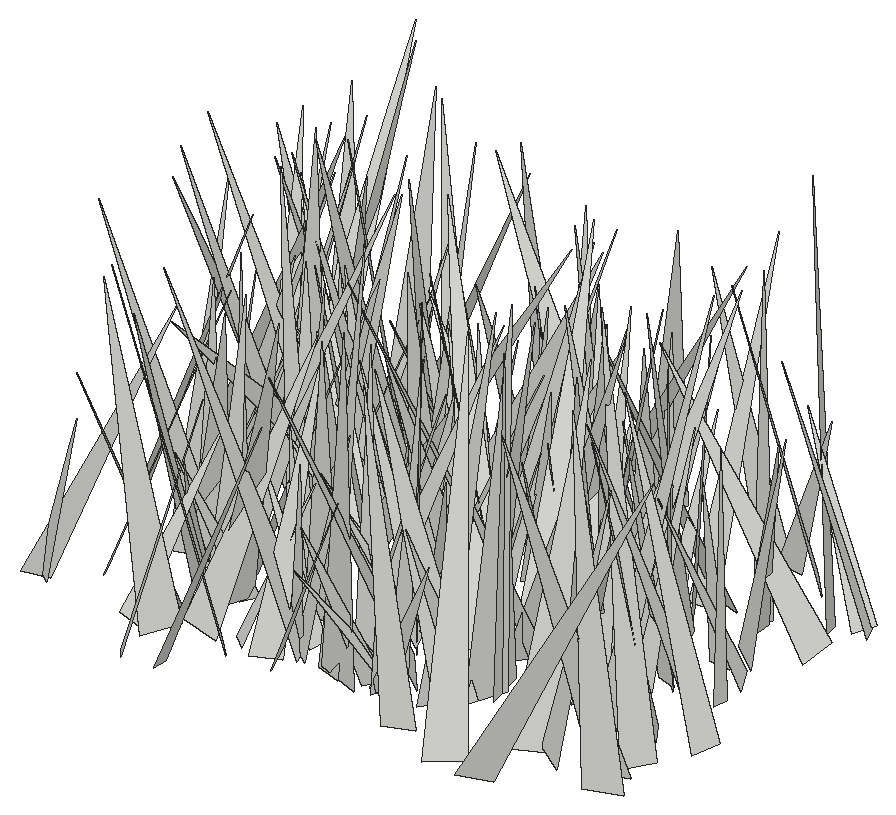
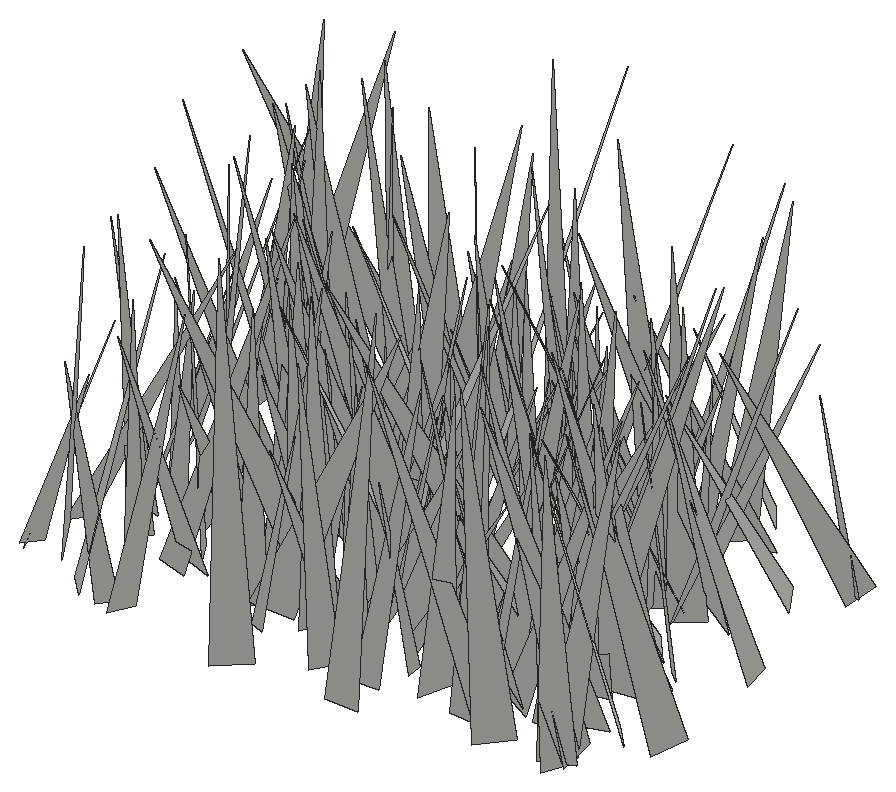
# SketchUp Ruby script. Lengths in inches.
U = 1.inch
M = Sketchup.active_model
def pt(a) = Geom::Point3d.new(a.map { |v| v * U })
def face(e, loops, mat)
  f = e.add_face(loops[0].map { |a| pt(a) })
  loops[1..].each { |l| e.add_face(l.map { |a| pt(a) }).erase! }
  f.material = f.back_material = mat if mat
  f
end
# faces: each face lists its corners as indices into pts; further lists are holes
def faces(e, pts, list, mat = nil) = list.each { |f| face(e, (f[0].is_a?(Array) ? f : [f]).map { |l| l.map { |i| pts[i] } }, mat) }
# xy, xz, yz: faces in a plane at the given z, y or x. An outline is a flat list of corners, or four numbers for a rectangle; further outlines are holes
def ring(l) = l.size == 4 ? [[l[0], l[1]], [l[2], l[1]], [l[2], l[3]], [l[0], l[3]]] : l.each_slice(2).to_a
def flat(e, list, mat, &to3) = list.each { |f| face(e, (f[0].is_a?(Array) ? f : [f]).map { |l| ring(l).map { |u, v| to3.(u, v) } }, mat) }
def xy(e, z, list, mat = nil) = flat(e, list, mat) { |x, y| [x, y, z] }
def xz(e, y, list, mat = nil) = flat(e, list, mat) { |x, z| [x, y, z] }
def yz(e, x, list, mat = nil) = flat(e, list, mat) { |y, z| [x, y, z] }
def lines(e, pts, list) = list.each { |a, b| e.add_line(pt(pts[a]), pt(pts[b])) }
# prism: a flat outline (further loops are holes) pulled along v
def prism(e, loops, v, mat = nil)
  f = face(e, loops, mat); d = Geom::Vector3d.new(v.map { |x| x * U })
  f.pushpull(f.normal.samedirection?(d) ? d.length : -d.length)
end
def box(e, o, s, mat = nil) = prism(e, [[o, [o[0] + s[0], o[1], o[2]], [o[0] + s[0], o[1] + s[1], o[2]], [o[0], o[1] + s[1], o[2]]]], [0, 0, s[2]], mat)
def at(x, y, z, deg = 0) = Geom::Transformation.translation(pt([x, y, z])) * Geom::Transformation.rotation(ORIGIN, Z_AXIS, deg.degrees)
def axes(o, x, y, z) = Geom::Transformation.new([*x, 0, *y, 0, *z, 0, *pt(o).to_a, 1])
def part(name) = M.definitions.add(name)
# library, detail: a bought-in or finely detailed component or shape, given as its bounding box
def library(name, o, s) = part(name).tap { |d| box(d.entities, o, s) }
def detail(e, o, s) = box(e.add_group.entities, o, s)
def put(e, d, t, mat = nil) = e.add_instance(d, t).tap { |i| i.material = mat if mat }
def group(e, t, mat = nil) = e.add_group.tap { |g| g.transformation = t; g.material = mat if mat }.entities
root = M.entities
c1 = part("fur_instance\#9")
p = [[0.8125,0,1.79],[0.67,-0.02,1.48],[0,-0.11,0],[0,0.11,0]]
faces(c1.entities,p,[[0,1,2,3]])
put(root,c1,axes([93.47,361.45,-27.1],[-5.98098,3.27291,2.42019],[3.72115,6.13978,0.89298],[1.64993,-1.98304,6.75918]))
put(root,c1,axes([94.98,359.49,-27.1],[4.77629,1.47467,0.59608],[1.29577,-4.70156,1.24867],[-0.92247,1.03128,4.84029]))
put(root,c1,axes([93.41,359.22,-27.1],[3.76197,3.17485,0.58422],[2.97684,-3.75885,1.25811],[-1.24876,0.60394,4.75913]))
put(root,c1,axes([102.43,364.67,-27.1],[-6.0329,-5.73941,0.68236],[-5.34499,5.91535,2.49841],[2.19943,-1.36753,7.94322]))
put(root,c1,axes([97.98,362.39,-27.1],[5.19096,1.17327,0.15724],[1.14991,-4.82989,-1.92283],[0.28108,-1.90867,4.96239]))
put(root,c1,axes([95.97,361.87,-27.1],[-5.67662,-5.13617,1.32256],[-5.29359,5.60645,-0.94818],[0.32758,1.59402,7.59639]))
put(root,c1,axes([108.84,360,-27.1],[6.56364,-3.25708,1.01889],[-3.38805,-5.95385,2.79299],[0.40967,2.94467,6.77415]))
put(root,c1,axes([100.55,362.6,-27.1],[-1.23371,-7.71978,2.49826],[-7.92295,1.69122,1.31342],[1.75022,2.21429,7.70662]))
put(root,c1,axes([104.48,361.15,-27.1],[-1.23354,6.12021,2.2306],[6.48252,0.93032,1.03231],[-0.63996,-2.37312,6.15735]))
put(root,c1,axes([102.16,363.6,-27.1],[-3.24466,-1.65637,0.06319],[-1.44148,2.88818,1.68993],[0.81834,-1.47993,3.2273]))
put(root,c1,axes([101.77,363.15,-27.1],[1.92833,-3.54748,0.58332],[-3.33012,-2.01195,-1.22706],[-1.35468,-0.10385,3.84674]))
put(root,c1,axes([112.54,363.17,-27.1],[0.14854,-7.36709,1.66817],[-7.40985,-0.46607,-1.39849],[-1.46661,1.60862,7.23466]))
put(root,c1,axes([87.66,361.98,-27.1],[2.1321,2.91958,1.28602],[3.18698,-1.87905,-1.01782],[0.14466,-1.63367,3.46899]))
put(root,c1,axes([102.47,362.65,-27.1],[1.15805,-3.96128,0.43832],[-3.70743,-0.90324,1.63219],[1.46246,0.84697,3.79062]))
put(root,c1,axes([113.02,362.05,-27.1],[1.15068,-6.84996,3.27998],[-7.48842,-1.57649,-0.66528],[-1.26644,3.09791,6.914]))
put(root,c1,axes([98.26,363.66,-27.1],[-7.76303,-2.55675,1.09489],[-2.43873,7.81802,0.96517],[1.33728,-0.58482,8.11604]))
put(root,c1,axes([93.29,362.93,-27.1],[-3.10953,-4.00727,0.37973],[-3.98696,3.00024,-0.98706],[-0.55366,0.90108,4.97525]))
put(root,c1,axes([102.33,362.84,-27.1],[3.31226,-1.52366,0.97308],[-1.49474,-3.45052,-0.31491],[-1.01694,0.10903,3.63228]))
put(root,c1,axes([107.26,360.28,-27.1],[5.53383,-2.65462,5.00816],[-4.23304,-6.59023,1.18414],[-3.76962,3.5034,6.0223]))
put(root,c1,axes([92.13,361.35,-27.1],[0.26684,4.21608,0.5662],[4.07293,-0.08948,-1.25314],[1.22767,-0.6195,4.03438]))
put(root,c1,axes([105.17,363.61,-27.1],[4.68158,-4.31782,3.21331],[-4.18207,-5.59908,-1.43065],[-3.3881,0.94493,6.20597]))
put(root,c1,axes([104.95,364.54,-27.1],[4.08531,-1.79648,1.28746],[-1.24322,-4.1049,-1.78292],[-1.82737,-1.22355,4.09124]))
put(root,c1,axes([93.17,364.28,-27.1],[-2.27159,-6.08211,1.19958],[-6.16809,2.34544,0.21162],[0.62109,1.04786,6.48903]))
put(root,c1,axes([110.01,362.77,-27.1],[3.01267,4.99828,1.819],[5.31773,-2.78497,-1.15474],[0.11548,-2.15148,5.72063]))
put(root,c1,axes([94.23,364.5,-27.1],[7.12513,-3.29011,0.44393],[-3.26274,-7.13377,-0.50321],[-0.6135,-0.27186,7.83192]))
put(root,c1,axes([98,363.45,-27.1],[-1.12295,-3.74744,1.45837],[-3.89173,1.39395,0.58526],[1.01223,1.20198,3.86805]))
put(root,c1,axes([94.55,362.3,-27.1],[0.24671,6.36494,1.6516],[6.30189,0.24313,-1.87833],[1.87786,-1.65213,6.08648]))
put(root,c1,axes([96.19,362.5,-27.1],[2.19151,2.85606,0.09461],[2.85445,-2.18225,-0.24214],[0.13471,-0.22234,3.59182]))
put(root,c1,axes([98.43,363.11,-27.1],[2.5994,3.80823,1.24151],[3.99906,-2.55122,-0.54734],[-0.2268,-1.33772,4.57819]))
put(root,c1,axes([87.5,361.79,-27.1],[5.30796,-1.91017,1.71118],[-2.50762,-4.68997,2.54311],[-0.53734,3.01775,5.03546]))
put(root,c1,axes([91.82,365.71,-27.1],[4.12034,-0.14152,0.59374],[0.17297,-3.61498,-2.06197],[-0.58535,-2.06437,3.57009]))
put(root,c1,axes([94.5625,365.13,-27.1],[1.61464,-3.26071,0.69447],[-2.99454,-1.75765,-1.29032],[-1.46534,-0.00102,3.40211]))
put(root,c1,axes([97.64,362.19,-27.1],[-4.32625,3.6169,1.13686],[3.35652,4.45591,-1.40339],[1.76301,0.39209,5.46158]))
put(root,c1,axes([98.51,364.06,-27.1],[-3.79909,0.62191,0.11225],[0.62576,3.79759,0.13861],[0.08831,-0.15497,3.84716]))
put(root,c1,axes([103.35,362.37,-27.1],[-6.05732,0.47074,1.68041],[-0.07648,5.99257,-1.95441],[1.74342,1.89841,5.75265]))
put(root,c1,axes([109.24,362.83,-27.1],[-4.71435,5.59524,2.23508],[5.56124,5.13291,-1.11952],[2.31839,-0.93486,7.23039]))
put(root,c1,axes([97.51,365.56,-27.1],[0.93072,-6.54849,1.55591],[-6.7031,-0.75944,0.81335],[0.60996,1.64631,6.5641]))
put(root,c1,axes([100.09,362.68,-27.1],[3.45024,7.01244,2.07893],[6.95776,-3.8555,1.45774],[-2.25516,-1.1667,7.67811]))
put(root,c1,axes([97.52,364.45,-27.1],[0.08392,3.77547,1.67654],[4.10941,-0.2474,0.35143],[-0.42151,-1.66031,3.76001]))
put(root,c1,axes([105.5625,364.77,-27.1],[7.52534,-2.11015,2.94691],[-2.32099,-8.02168,0.183],[-2.78389,0.98374,7.81345]))
put(root,c1,axes([104.37,363.28,-27.1],[-6.74927,1.80081,2.69667],[1.18797,7.16726,-1.81295],[3.01723,1.2063,6.74602]))
put(root,c1,axes([105.72,365.63,-27.1],[-6.42267,-1.42598,3.31634],[-1.29179,7.22813,0.60623],[3.37087,0.05298,6.55107]))
put(root,c1,axes([91.19,367.07,-27.1],[3.73638,-5.69312,0.32255],[-5.69521,-3.70663,0.54933],[0.28337,0.57053,6.78752]))
put(root,c1,axes([101.1,366.62,-27.1],[-3.84083,-1.16764,0.10273],[-1.10793,3.73134,0.98769],[0.38264,-0.91633,3.89099]))
put(root,c1,axes([104.73,365.6,-27.1],[7.78387,0.2727,2.09642],[0.3333,-8.05673,-0.18953],[-2.08764,-0.26953,7.78634]))
put(root,c1,axes([100.16,364.73,-27.1],[1.00537,5.49165,1.69021],[5.63183,-1.28199,0.81538],[-1.13911,-1.49133,5.52306]))
put(root,c1,axes([101.02,366.47,-27.1],[5.50119,4.10651,2.99111],[4.73487,-5.74232,-0.82461],[-1.84151,-2.49711,6.81516]))
put(root,c1,axes([89.3,363.54,-27.1],[4.7893,3.01055,0.30481],[2.77693,-4.59952,1.79634],[-1.20208,1.36921,5.36414]))
put(root,c1,axes([93.03,365.52,-27.1],[4.88657,-1.90502,2.44295],[-2.30886,-5.28158,0.49977],[-2.06549,1.39696,5.22091]))
put(root,c1,axes([111.91,366.53,-27.1],[-4.7875,-3.33897,1.34753],[-3.4677,4.87923,-0.23006],[0.96934,0.96392,5.83232]))
put(root,c1,axes([91.79,366.2,-27.1],[0.33576,5.45677,2.6197],[6.05197,-0.25349,-0.24764],[0.11336,-2.62894,5.46148]))
put(root,c1,axes([91.74,366.74,-27.1],[-7.05109,-1.52018,0.70264],[-1.52291,7.08527,0.04653],[0.69669,0.10238,7.21295]))
put(root,c1,axes([99.61,367.9,-27.1],[-4.59032,-0.23962,0.17171],[-0.16134,4.28449,1.66587],[0.24672,-1.65642,4.28408]))
put(root,c1,axes([113.07,367.71,-27.1],[-6.09562,-2.74651,0.83103],[-2.67616,6.14538,0.68045],[1.03541,-0.28555,6.65108]))
put(root,c1,axes([112.82,364.31,-27.1],[-8.1921,1.36867,0.61461],[1.20152,8.02801,-1.8625],[0.89853,1.74336,8.09413]))
put(root,c1,axes([105.68,367.79,-27.1],[-0.21744,-4.53269,0.61909],[-4.46943,0.07824,-0.99696],[-0.9761,0.65149,4.42703]))
put(root,c1,axes([92.64,366.91,-27.1],[0.05129,-4.93553,2.34933],[-4.99892,0.90807,2.01684],[2.21125,2.16734,4.50493]))
put(root,c1,axes([99.3125,365.72,-27.1],[3.76049,3.04894,0.61025],[2.98388,-3.80785,0.6375],[-0.87456,0.11813,4.79905]))
put(root,c1,axes([99.18,366.15,-27.1],[3.55811,5.92159,0.8478],[5.93377,-3.36884,-1.37307],[0.75783,-1.4247,6.77052]))
put(root,c1,axes([105.36,370.32,-27.1],[1.43301,-8.2393,0.15598],[-8.02359,-1.35888,1.93375],[1.87948,0.48092,8.13635]))
put(root,c1,axes([113.97,366.72,-27.1],[-6.67851,0.63047,0.27765],[0.60623,6.66388,-0.54986],[0.32721,0.52189,6.68563]))
put(root,c1,axes([92.96,366.58,-27.1],[-5.66532,-0.50223,1.85308],[-0.88322,5.80808,-1.12609],[1.70472,1.34012,5.57494]))
put(root,c1,axes([93.61,366.39,-27.1],[4.63443,1.21877,0.59299],[1.09033,-4.6073,0.94811],[-0.80513,0.77609,4.69728]))
put(root,c1,axes([104.89,367.86,-27.1],[7.07738,-3.29601,0.99897],[-3.4049,-7.03943,0.89669],[-0.51794,1.23844,7.75557]))
put(root,c1,axes([100.48,367.1875,-27.1],[5.45999,3.37552,0.2587],[3.37248,-5.38033,-0.97518],[0.29572,-0.96459,6.34466]))
put(root,c1,axes([106.65,369.62,-27.1],[1.50872,-5.62418,0.24688],[-5.60162,-1.47433,0.64555],[0.56049,0.40439,5.78713]))
put(root,c1,axes([99.46,369.71,-27.1],[-0.15941,-4.26775,0.08772],[-3.87813,0.18147,1.78158],[1.78369,0.01316,3.88138]))
put(root,c1,axes([100.71,369.86,-27.1],[1.73584,-5.70606,0.92261],[-5.63591,-1.88469,-1.0526],[-1.28332,0.55882,5.87063]))
put(root,c1,axes([110.05,365.88,-27.1],[3.85814,7.37241,1.12129],[7.37277,-3.96052,0.67189],[-1.11889,-0.67587,8.29374]))
put(root,c1,axes([101.55,371.1,-27.1],[-5.30348,-5.59312,0.1785],[-5.55783,5.29332,0.73008],[0.65218,-0.37354,7.67313]))
put(root,c1,axes([95.92,366.49,-27.1],[-7.72963,0.57294,0.92033],[0.30078,7.49944,-2.14251],[1.04153,2.08628,7.44883]))
put(root,c1,axes([99.85,368.17,-27.1],[-4.67921,0.76999,0.1435],[0.76372,4.67821,-0.1991],[0.17382,0.17327,4.73796]))
put(root,c1,axes([108.08,366.82,-27.1],[6.4621,3.38539,1.99868],[3.00841,-6.73382,1.67909],[-2.53082,0.63956,7.09931]))
put(root,c1,axes([91.97,366.47,-27.1],[4.66085,6.54813,0.11631],[6.5407,-4.64683,-0.4912],[0.3329,-0.37945,8.02249]))
put(root,c1,axes([93.57,373.72,-27.1],[5.32765,-5.22538,0.29084],[-4.03169,-4.36253,-4.52625],[-3.33686,-3.07194,5.93309]))
put(root,c1,axes([90.4375,366.25,-27.1],[2.16067,6.65454,0.44246],[6.23565,-2.18071,2.34697],[-2.36543,0.32979,6.59114]))
put(root,c1,axes([103.35,367.72,-27.1],[-5.00695,6.61488,0.9269],[6.67749,4.92855,0.89773],[-0.16413,-1.27989,8.24744]))
put(root,c1,axes([86.73,368.69,-27.1],[6.39935,1.66924,0.57136],[1.67346,-6.42366,0.02366],[-0.55885,-0.12123,6.61343]))
put(root,c1,axes([94.04,370.78,-27.1],[1.95757,-4.55386,0.31612],[-4.56359,-1.94437,0.25034],[0.10577,0.38911,4.95045]))
put(root,c1,axes([102.51,368.68,-27.1],[-0.54447,5.56352,1.73211],[5.79599,0.33809,0.73596],[-0.59958,-1.78391,5.54144]))
put(root,c1,axes([109.8125,369.67,-27.1],[-2.15143,-4.58063,1.63472],[-4.86135,2.07952,-0.57094],[0.14745,1.72526,5.02841]))
put(root,c1,axes([104.61,369.92,-27.1],[-1.9321,-3.03286,0.9193],[-3.13143,1.99261,-0.00754],[0.48737,0.77951,3.596]))
put(root,c1,axes([101.43,370.35,-27.1],[3.99613,2.0991,0.80323],[2.24013,-3.58697,-1.77087],[0.18236,-1.93595,4.15203]))
put(root,c1,axes([109.92,369.8,-27.1],[4.37424,4.04681,2.79179],[4.54542,-4.75288,-0.23239],[-1.87347,-2.08284,5.95454]))
put(root,c1,axes([92.67,370.76,-27.1],[-7.47727,-2.4998,1.10622],[-2.44373,7.5564,0.55783],[1.22512,-0.18436,7.86431]))
put(root,c1,axes([103.01,368.05,-27.1],[-1.19348,5.65379,0.3473],[5.3271,0.99964,2.033],[-1.92561,-0.73875,5.40894]))
put(root,c1,axes([111.91,371.4375,-27.1],[-4.09527,-2.1175,0.66115],[-1.87882,4.04889,1.32991],[1.17939,-0.90267,4.41434]))
put(root,c1,axes([93.14,370.04,-27.1],[5.23095,-0.44242,1.6949],[-0.413,-5.49862,-0.16069],[-1.70231,-0.02548,5.24716]))
put(root,c1,axes([90.93,372.87,-27.1],[-1.44964,-7.72306,0.36058],[-7.72764,1.4358,-0.315],[-0.24346,0.41228,7.85162]))
put(root,c1,axes([89.07,370.45,-27.1],[3.62429,3.41254,1.71474],[3.78655,-3.51895,-1.00013],[-0.49783,-1.92166,4.87654]))
put(root,c1,axes([105.39,372.28,-27.1],[5.27759,-3.33069,0.22963],[-3.2336,-5.20637,-1.19863],[-0.83073,-0.89406,6.12452]))
put(root,c1,axes([96.05,370.08,-27.1],[-3.65286,-4.07637,1.60167],[-4.37583,3.48496,-1.11027],[0.18514,1.94004,5.3598]))
put(root,c1,axes([107.84,368.02,-27.1],[0.68594,6.83231,0.78357],[6.74689,-0.82108,1.2531],[-1.33188,-0.64057,6.75135]))
put(root,c1,axes([109.4,368.83,-27.1],[1.25627,4.75609,0.70963],[4.78282,-1.31187,0.32531],[-0.49861,-0.60066,4.90844]))
put(root,c1,axes([104.28,370.94,-27.1],[-2.25784,-3.06403,1.232],[-3.11024,2.47464,0.4545],[1.1102,0.70132,3.77883]))
put(root,c1,axes([100.89,371.24,-27.1],[3.77255,3.78798,3.73229],[4.48771,-4.72284,0.25719],[-2.85294,-2.4201,5.33992]))
put(root,c1,axes([105.02,368.31,-27.1],[-3.53884,7.24303,1.02774],[7.25201,3.62348,-0.56563],[0.96238,-0.67082,8.04145]))
put(root,c1,axes([97.62,370.875,-27.1],[2.40925,-3.29701,1.00546],[-3.44676,-2.29271,0.74099],[0.03277,1.24857,4.01568]))
put(root,c1,axes([112.3,369.625,-27.1],[-4.48133,-0.60292,1.35721],[-0.97091,4.45413,-1.22715],[1.12377,1.44397,4.35201]))
put(root,c1,axes([104.21,372.39,-27.1],[6.83248,-2.68093,1.04491],[-2.55055,-6.88917,-0.99801],[-1.33189,-0.56029,7.27146]))
put(root,c1,axes([100.55,371.02,-27.1],[-3.18222,-1.83698,0.96818],[-1.93012,3.2701,-0.13938],[0.76583,0.60852,3.67173]))
put(root,c1,axes([94.68,368.36,-27.1],[4.61652,6.22378,1.13894],[6.03614,-4.75491,1.51682],[-1.89675,0.0163,7.59914]))
put(root,c1,axes([108.72,372.25,-27.1],[-6.30807,-3.21691,2.7037],[-2.95993,6.86307,1.25992],[2.98285,0.00727,6.96799]))
put(root,c1,axes([101.82,372.33,-27.1],[2.32363,-4.81619,0.47979],[-4.81966,-2.25368,0.71896],[0.44354,0.74187,5.29887]))
put(root,c1,axes([90.77,369.04,-27.1],[3.00596,2.69315,0.13963],[2.45938,-2.82346,1.51258],[-1.10635,1.04086,3.74179]))
put(root,c1,axes([110.53,371.82,-27.1],[0.0054,-4.02258,1.09842],[-4.16704,0.03516,0.14925],[0.15324,1.09787,4.01982]))
put(root,c1,axes([103.375,370.84,-27.1],[3.80415,1.70942,1.42934],[1.7089,-4.05302,0.29902],[-1.42996,-0.29602,4.15984]))
put(root,c1,axes([106.6,369.83,-27.1],[-4.20959,5.12778,0.85898],[5.1677,4.24809,-0.03415],[0.57165,-0.64206,6.63427]))
put(root,c1,axes([105.72,372.08,-27.1],[0.0044,-6.27087,2.13822],[-6.5778,-0.25997,-0.7489],[-0.79272,2.12236,6.226]))
put(root,c1,axes([99.6875,372.2,-27.1],[2.95462,-6.48005,1.02046],[-5.97059,-2.19282,3.36242],[2.71745,2.2277,6.27814]))
put(root,c1,axes([101.51,370.4,-27.1],[2.79902,6.82497,1.56007],[7.00009,-2.70115,-0.74237],[0.11309,-1.72399,7.33919]))
put(root,c1,axes([106.88,369.95,-27.1],[1.72672,7.47142,1.23195],[7.48463,-1.49226,-1.44043],[1.14896,-1.50745,7.53186]))
put(root,c1,axes([96.29,373.02,-27.1],[4.8862,-3.80667,1.31151],[-3.74132,-5.05482,-0.73291],[-1.48774,0.20937,6.1505]))
put(root,c1,axes([105.53,370.1875,-27.1],[-3.3116,2.69695,0.72945],[2.42136,3.33487,-1.33716],[1.39378,0.61437,4.05614]))
put(root,c1,axes([91.51,371.96,-27.1],[2.46407,-3.91283,1.91735],[-4.25122,-2.64198,0.07181],[-0.95581,1.66367,4.6235]))
put(root,c1,axes([93.38,372.15,-27.1],[-7.85705,-0.88135,0.16267],[-0.88597,7.85465,-0.23661],[0.1352,0.25331,7.90278]))
put(root,c1,axes([88.35,371.54,-27.1],[3.49532,2.40186,0.16337],[2.40303,-3.46356,-0.49202],[0.14512,-0.49771,4.21237]))
put(root,c1,axes([92.17,372.52,-27.1],[1.0853,-7.02468,2.48253],[-7.23303,-0.3918,2.05344],[1.78669,2.68091,6.80495]))
put(root,c1,axes([110.92,372.73,-27.1],[-1.89095,-4.65132,2.366],[-4.60338,2.67208,1.57395],[2.45798,1.42605,4.76793]))
put(root,c1,axes([96.24,371.9,-27.1],[-6.99068,-2.50094,0.47101],[-2.54423,6.83653,-1.46112],[-0.05835,1.53405,7.27938]))
put(root,c1,axes([87.7,372.99,-27.1],[1.22983,-5.08709,1.30795],[-5.046,-0.77126,1.74491],[1.45845,1.62123,4.93419]))
put(root,c1,axes([95.33,370.94,-27.1],[7.21653,-2.33327,0.39687],[-2.31249,-6.67999,2.77668],[0.50399,2.75925,7.05779]))
put(root,c1,axes([90.52,373.34,-27.1],[1.05516,-7.50337,2.43147],[-7.87164,-0.84629,0.8044],[0.49989,2.51181,7.53438]))
put(root,c1,axes([90.88,369.06,-27.1],[4.07419,5.57288,0.07978],[5.18286,-3.82462,2.48447],[-2.04971,1.40628,6.44076]))
put(root,c1,axes([94.53,371.1875,-27.1],[-3.04335,5.85133,0.32291],[5.70958,2.87864,1.64877],[-1.32023,-1.03909,6.38604]))
put(root,c1,axes([110.125,374.35,-27.1],[5.73315,-1.08828,0.33068],[-0.98004,-5.58896,-1.40205],[-0.57725,-1.3198,5.66459]))
put(root,c1,axes([107.92,375.375,-27.1],[-1.99035,-6.59495,0.1128],[-6.59501,1.99173,0.07994],[0.10913,0.08488,6.88828]))
put(root,c1,axes([97.71,373.03,-27.1],[4.40599,-6.63506,1.39046],[-6.52465,-3.70025,3.01783],[1.84021,2.76664,7.37085]))
put(root,c1,axes([92.23,371.22,-27.1],[-0.89857,4.82904,0.37817],[4.8418,0.88433,0.21213],[-0.14006,-0.41036,4.90735]))
put(root,c1,axes([93.55,373.39,-27.1],[3.00214,-3.52749,1.91618],[-3.65397,-3.39209,-0.51969],[-1.66236,1.08552,4.60282]))
put(root,c1,axes([106.88,371.78,-27.1],[2.68485,5.08236,0.90598],[5.15716,-2.6868,-0.21076],[-0.23424,-0.9002,5.74408]))
put(root,c1,axes([87.57,372.91,-27.1],[5.01329,4.55618,1.17415],[4.70331,-4.80639,-1.43108],[0.12753,-1.84671,6.62147]))
put(root,c1,axes([100.75,370.55,-27.1],[4.99959,5.18328,0.38062],[5.01525,-4.9501,1.53324],[-1.36326,0.79826,7.03643]))
put(root,c1,axes([108.39,371.2,-27.1],[-3.90191,2.21296,0.38649],[1.88444,3.64598,-1.85127],[1.22289,1.44261,4.08594]))
put(root,c1,axes([100.03,373.875,-27.1],[-1.04898,-5.12431,2.12616],[-5.35306,1.50327,0.98203],[1.45734,1.83333,5.13756]))
put(root,c1,axes([112.7,374.62,-27.1],[-6.59727,0.97904,0.29915],[1.02311,6.37288,1.70633],[0.03533,-1.73199,6.44755]))
put(root,c1,axes([103.26,373.75,-27.1],[2.23095,-4.80055,1.901],[-5.14348,-2.24733,0.36107],[-0.45138,1.8816,5.28129]))
put(root,c1,axes([93.06,375.36,-27.1],[-0.40917,-7.70862,1.45343],[-7.84037,0.35495,-0.32469],[-0.25296,1.46762,7.71264]))
put(root,c1,axes([107.66,373.88,-27.1],[5.0794,2.90769,2.21904],[3.29641,-5.28463,-0.62087],[-1.58507,-1.67247,5.81975]))
put(root,c1,axes([103.52,372.11,-27.1],[-5.59441,-0.96055,0.72122],[-1.15543,5.24244,-1.98041],[0.32833,2.08191,5.31959]))
put(root,c1,axes([100.04,373.57,-27.1],[-3.98181,3.20015,0.16473],[3.12043,3.81261,1.36007],[-0.7287,-1.16015,4.92402]))
put(root,c1,axes([99.5625,373.21,-27.1],[-5.02924,-0.94611,0.83871],[-1.10156,4.96734,-1.00192],[0.62059,1.14984,5.01842]))
put(root,c1,axes([89.83,372.61,-27.1],[-1.61925,6.67608,1.38838],[6.8184,1.60284,0.24489],[0.08425,-1.4073,6.86528]))
put(root,c1,axes([89.64,371.75,-27.1],[2.76869,6.15296,0.77217],[6.00563,-2.8712,1.34513],[-1.54517,-0.13446,6.61174]))
put(root,c1,axes([104.3,373.72,-27.1],[1.80379,6.11401,2.80003],[6.29213,-2.55743,1.53087],[-2.37284,-2.13386,6.18799]))
put(root,c1,axes([97.13,371.58,-27.1],[3.53249,6.50702,1.2231],[6.07163,-3.73652,2.34297],[-2.64057,0.11331,7.02355]))
put(root,c1,axes([85.97,374.58,-27.1],[7.43524,-1.67911,0.29476],[-1.69435,-7.42416,0.44731],[-0.18841,0.50147,7.60934]))
put(root,c1,axes([90.39,376.13,-27.1],[-0.97227,-5.54065,0.71566],[-5.53732,1.05209,0.62249],[0.741,0.5921,5.59077]))
put(root,c1,axes([99.91,374.98,-27.1],[4.11916,-1.93041,1.42636],[-1.9279,-4.34864,-0.31782],[-1.42975,0.30221,4.53795]))
put(root,c1,axes([96.21,374.99,-27.1],[1.60844,-3.68609,1.55705],[-3.78668,-1.94455,-0.69177],[-1.29334,1.10916,3.96179]))
put(root,c1,axes([97.53,374.87,-27.1],[-2.45268,-3.25533,0.28731],[-3.08329,2.18606,-1.55237],[-1.08306,1.14864,3.76868]))
put(root,c1,axes([103.95,375.74,-27.1],[4.8037,-2.51399,0.9877],[-2.43404,-4.90267,-0.64073],[-1.17095,-0.12226,5.38379]))
put(root,c1,axes([92.3125,372.8,-27.1],[3.84867,2.11329,0.22175],[1.92609,-3.66331,1.48248],[-0.8974,1.20066,4.13285]))
put(root,c1,axes([92.2,375.54,-27.1],[-2.37076,-5.83706,1.32394],[-5.9146,2.06646,-1.48049],[-0.91737,1.76156,6.12372]))
put(root,c1,axes([101.71,374.19,-27.1],[7.5928,-1.32868,0.07278],[-1.31152,-7.40102,1.71058],[0.22497,1.69728,7.51598]))
put(root,c1,axes([93.06,375.93,-27.1],[-4.49464,-4.79472,1.8462],[-5.03521,4.59856,-0.3156],[1.02201,1.56958,6.56442]))
put(root,c1,axes([105.22,375.17,-27.1],[4.42317,-1.03576,2.17466],[-1.28949,-4.85884,0.30856],[-2.03449,0.82776,4.53233]))
put(root,c1,axes([93.09,377.48,-27.1],[-1.97553,-6.78705,1.45707],[-6.65434,2.28292,1.61176],[1.97656,0.90224,6.88251]))
put(root,c1,axes([101.17,375.45,-27.1],[-5.47966,3.19166,2.7493],[3.39794,6.01513,-0.2105],[2.48986,-1.18473,6.33791]))
put(root,c1,axes([94.47,373.64,-27.1],[2.91558,3.30379,0.88214],[2.68077,-2.92801,2.10571],[-2.12289,0.83996,3.8706]))
put(root,c1,axes([97.2,377.77,-27.1],[-0.08674,-5.50292,0.32115],[-5.49794,0.10952,0.39174],[0.3974,0.31411,5.48965]))
put(root,c1,axes([102.82,376.92,-27.1],[-1.51621,-3.26203,0.55212],[-3.23761,1.58793,0.49084],[0.68086,0.28668,3.56354]))
put(root,c1,axes([96.5,375.88,-27.1],[3.55375,0.65284,0.74182],[0.70307,-3.6162,-0.18565],[-0.69441,-0.32026,3.60844]))
put(root,c1,axes([92.18,375.4375,-27.1],[2.56604,4.25646,1.10853],[4.39439,-2.42581,-0.85772],[0.18887,-1.38883,4.89555]))
put(root,c1,axes([103.17,375.64,-27.1],[-4.31341,6.46311,1.11663],[6.32564,3.74609,2.75266],[-1.73345,-2.41229,7.26637]))
put(root,c1,axes([89.99,376.07,-27.1],[-3.27969,0.65416,1.38528],[0.68941,3.5533,-0.04576],[1.36808,-0.22237,3.34398]))
put(root,c1,axes([101.04,374.75,-27.1],[4.03542,0.28371,1.50858],[-0.2798,-4.0361,1.5075],[-1.50932,1.50677,3.754]))
put(root,c1,axes([87.81,374.97,-27.1],[4.5925,4.65986,1.11021],[4.70947,-4.6734,0.13435],[-0.87619,-0.69491,6.5412]))
put(root,c1,axes([88.76,377.4,-27.1],[3.4747,-4.84053,2.29693],[-4.84614,-4.00697,-1.11322],[-2.28507,1.13736,5.85363]))
put(root,c1,axes([109.89,375.05,-27.1],[-6.28866,-0.36775,1.68536],[-0.82762,6.23312,-1.72806],[1.51351,1.8804,6.05775]))
put(root,c1,axes([113.26,376.92,-27.1],[-4.74174,-2.50609,0.51828],[-2.55748,4.67952,-0.77105],[0.09149,0.92453,5.30754]))
put(root,c1,axes([99.17,377.64,-27.1],[4.9839,-2.53795,0.76874],[-2.53211,-5.04073,-0.2255],[-0.78777,0.14572,5.58834]))
put(root,c1,axes([88.23,378.3125,-27.1],[6.05752,-0.57817,0.88939],[-0.39,-6.0087,-1.2499],[-0.9865,-1.17476,5.9553]))
put(root,c1,axes([109.7,378.53,-27.1],[-4.76298,-4.61729,1.21885],[-4.61962,4.89113,0.47635],[1.20999,0.49843,6.61653]))
put(root,c1,axes([112.93,377,-27.1],[-3.82314,1.91513,0.41484],[1.95484,3.79049,0.51675],[0.13566,-0.64863,4.24466]))
put(root,c1,axes([91.85,377.38,-27.1],[7.09843,0.26187,0.16049],[0.26265,-7.10014,-0.03187],[-0.15921,-0.03777,7.10319]))
put(root,c1,axes([94.99,376.49,-27.1],[-6.58758,2.43197,1.48528],[2.355,6.75255,-0.6115],[1.60454,0.07391,6.99549]))
put(root,c1,axes([107.4,374.75,-27.1],[1.20703,6.81999,0.05967],[6.70849,-1.19813,1.23829],[-1.22962,0.158,6.81439]))
put(root,c1,axes([89.15,375.23,-27.1],[-1.14842,8.02715,0.79991],[8.02073,1.22255,-0.75306],[0.86188,-0.68125,8.07384]))
put(root,c1,axes([101.82,379.58,-27.1],[5.04429,-5.44094,0.7168],[-5.46997,-5.06343,0.05905],[-0.44381,0.56596,7.41924]))
put(root,c1,axes([88.16,377.07,-27.1],[7.83085,1.1219,1.78667],[1.00117,-8.02181,0.64907],[-1.85702,0.40616,7.88414]))
put(root,c1,axes([108.1,378.8,-27.1],[1.41621,-4.16021,0.5332],[-4.01988,-1.18575,1.42542],[1.19673,0.94019,4.15706]))
put(root,c1,axes([96.97,379.42,-27.1],[-0.69172,-7.26259,1.83893],[-7.46362,0.82804,0.46276],[0.64909,1.78171,7.28077]))
put(root,c1,axes([107.41,378.85,-27.1],[-5.83631,0.9789,1.84731],[1.28037,6.00401,0.86359],[1.65271,-1.19453,5.85448]))
put(root,c1,axes([112.05,376.22,-27.1],[-7.32928,-2.99407,2.48715],[-3.76161,6.81126,-2.88543],[1.00033,3.67572,7.37273]))
put(root,c1,axes([88.4,377.92,-27.1],[-2.28357,5.70644,2.33564],[6.0895,2.47813,-0.10083],[0.96778,-2.12809,6.14557]))
put(root,c1,axes([91.07,378.14,-27.1],[4.75602,-4.66812,2.75377],[-5.20371,-4.95731,0.58378],[-1.51526,2.37234,6.63855]))
